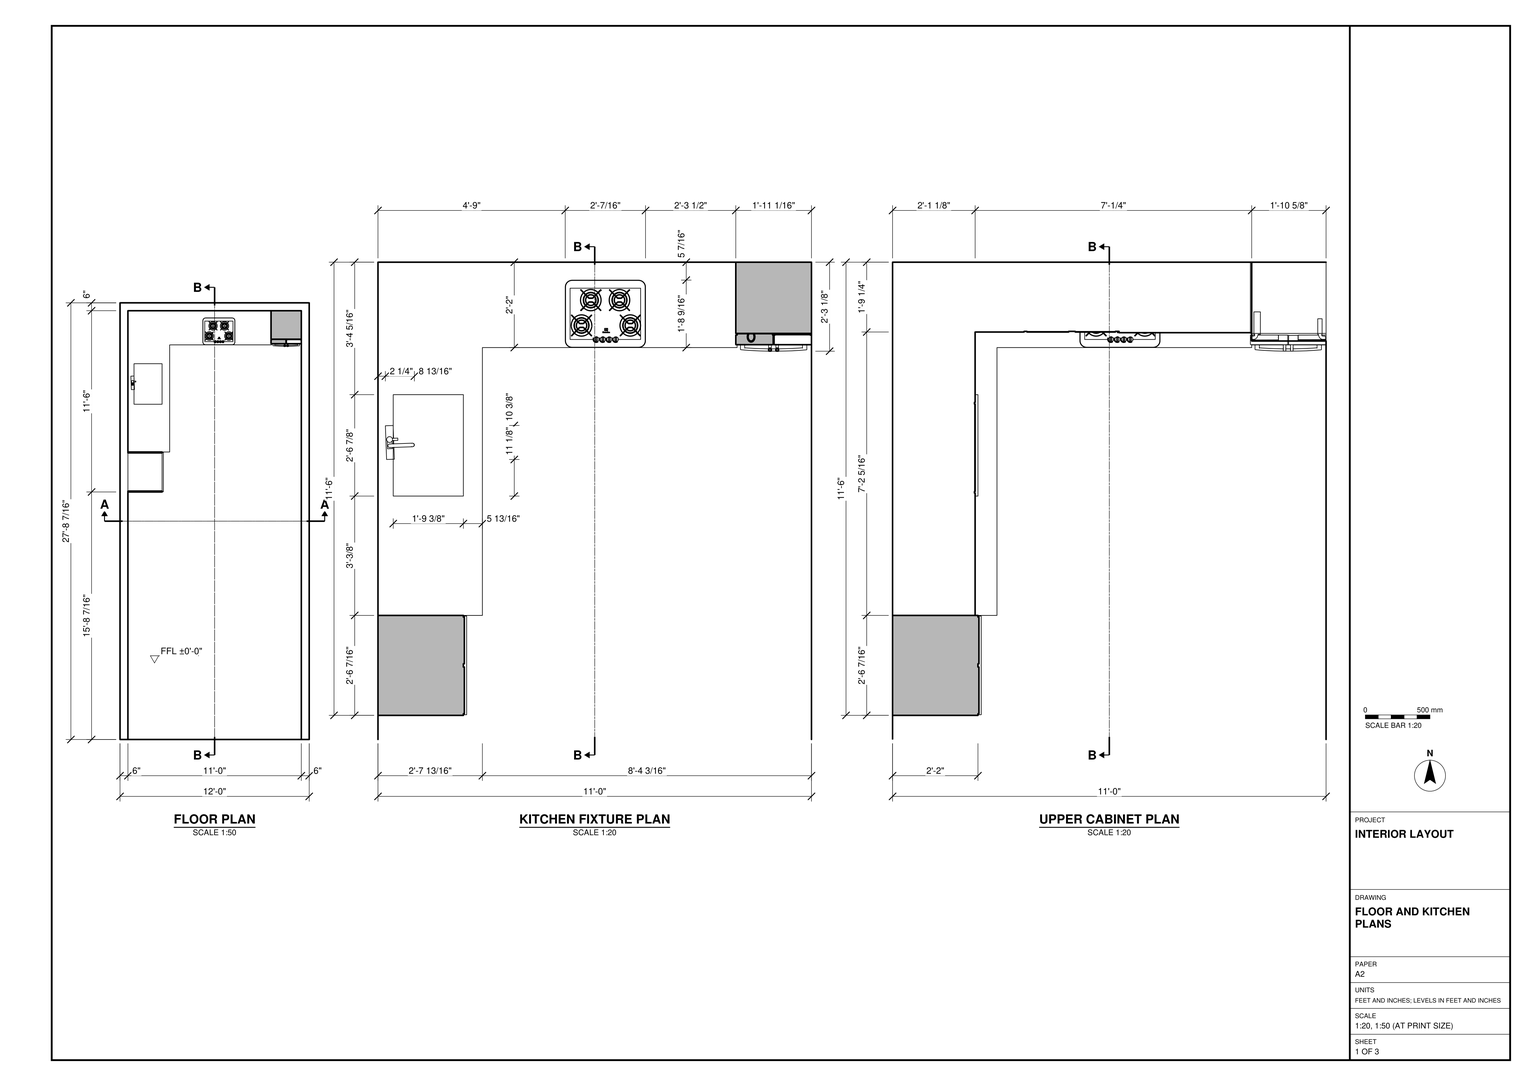
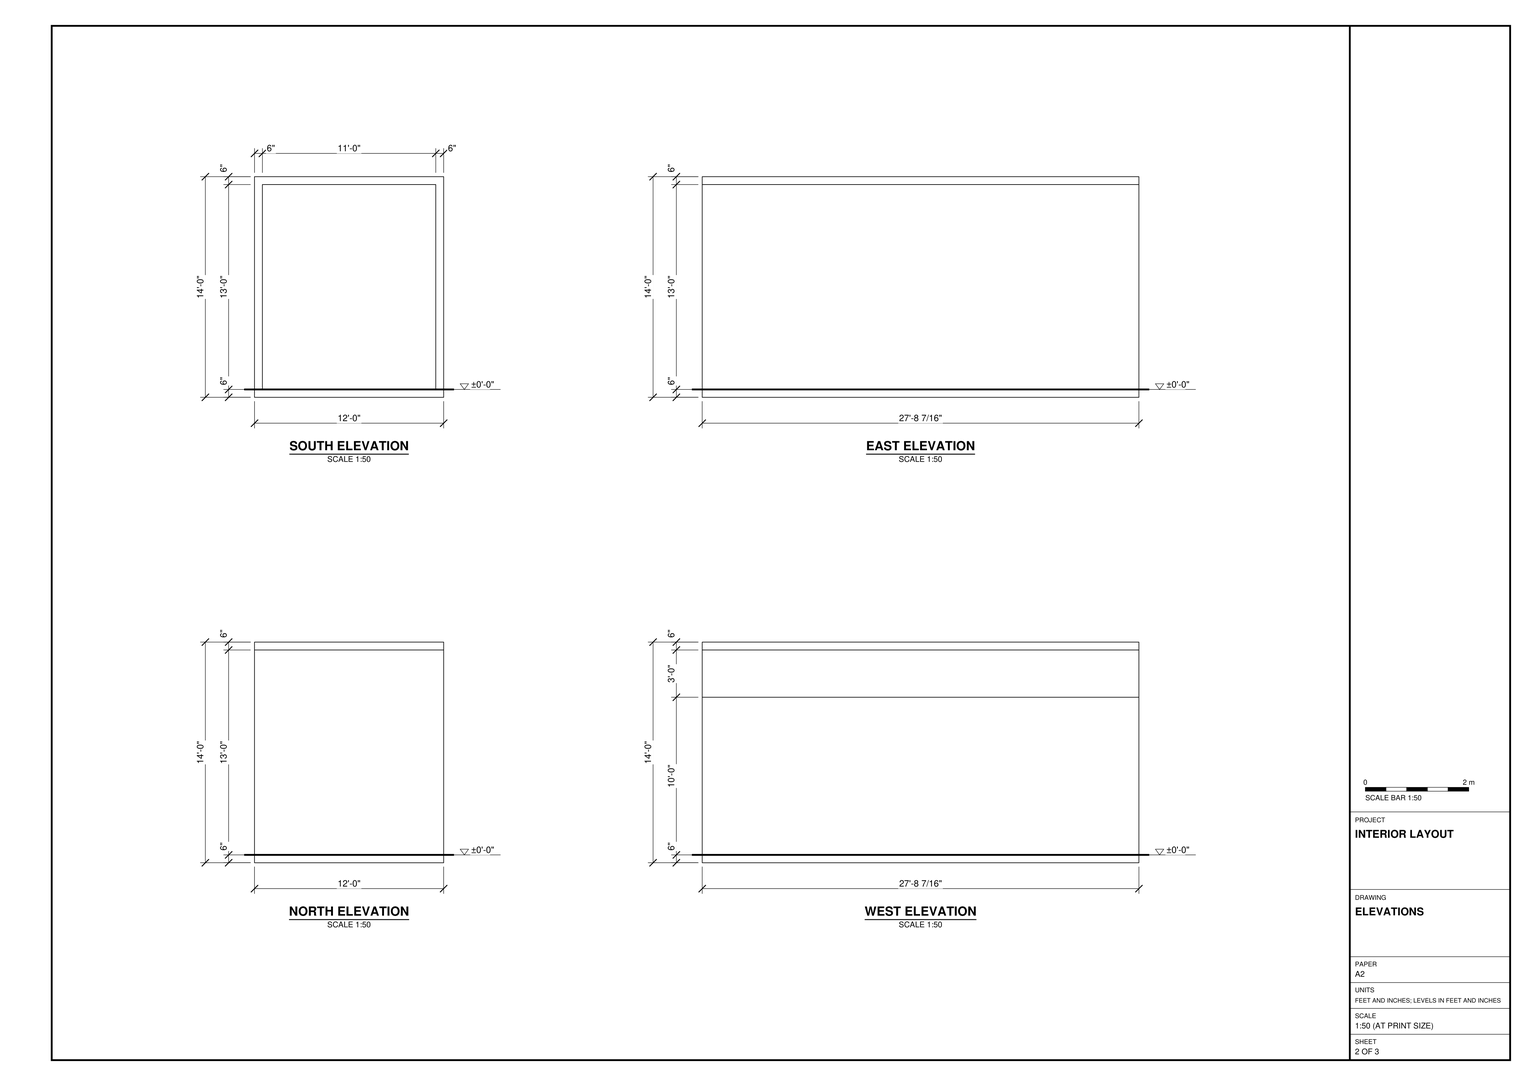
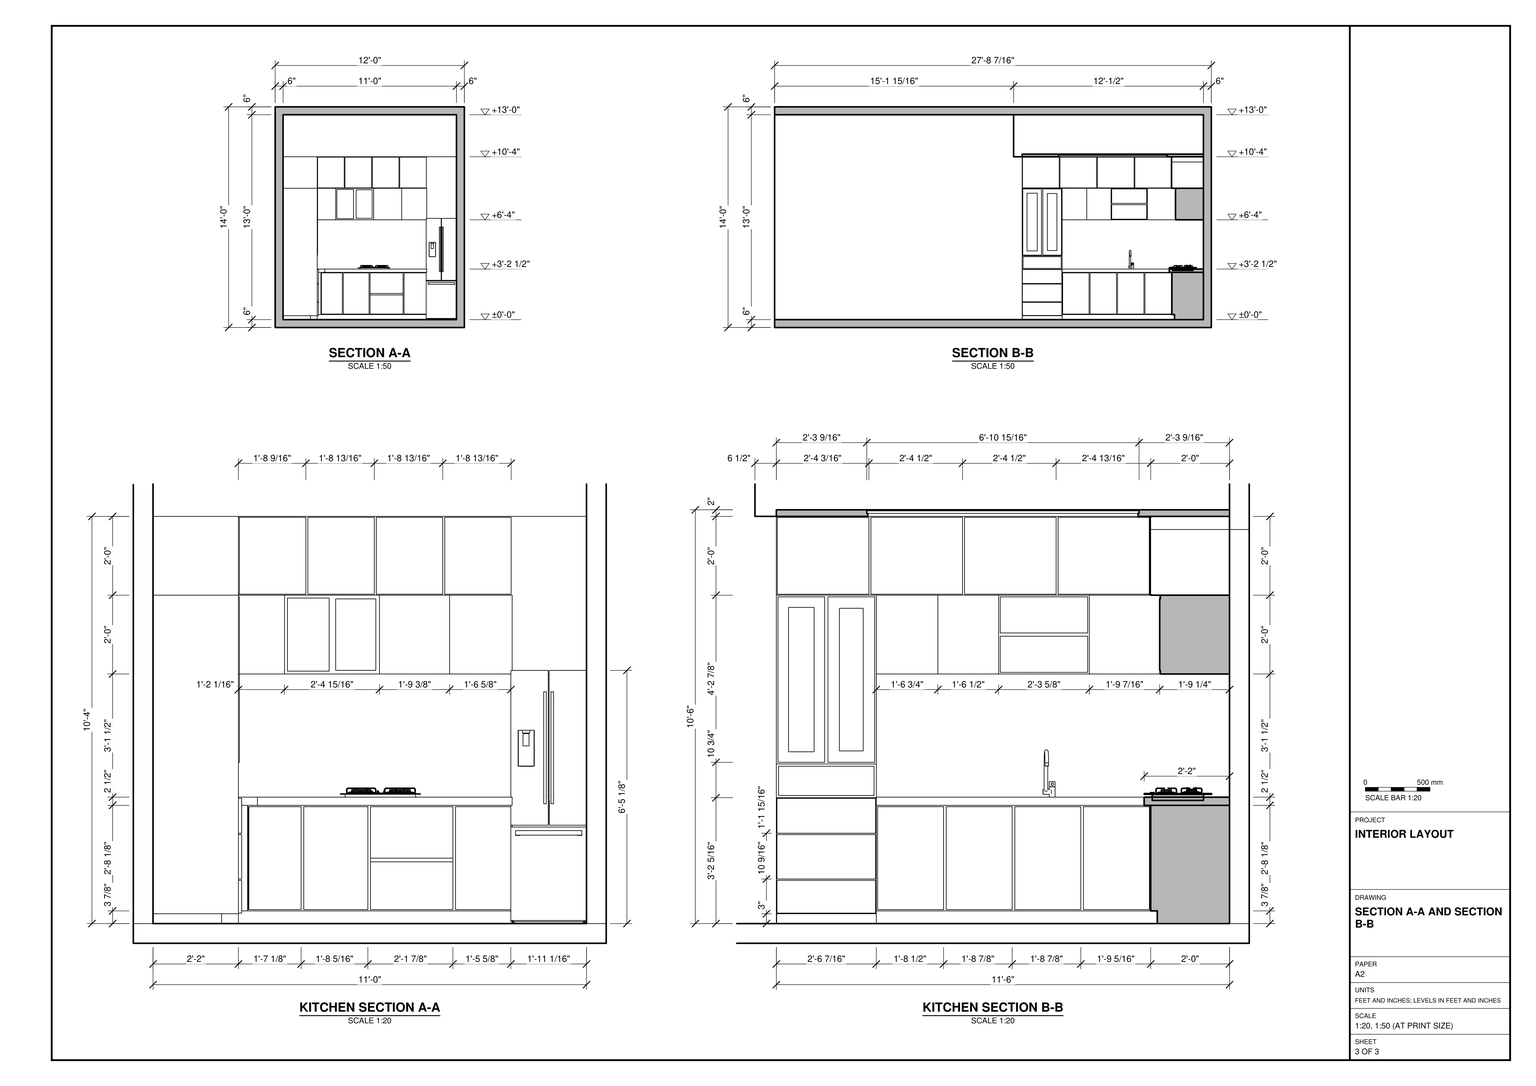
Build the interior in SketchUp using task_files/diagram_01.pdf. Work in feet and inches. Make the shell 12'-0" wide, 27'-8 7/16" long and 14'-0" high, with the finished floor at ±0'-0". Model the 6" side and north walls, the floor slab and the flat roof slab. Leave the south end open between the side walls, as shown in the floor plan and south elevation.

Fit the kitchen across the north end and along the west wall, leaving the floor to the south clear. Use the fixture plan to set out the worktop depths, the sink and tap on the west run, the cooktop on the north run and the refrigerator at the east end. Finish the west run with the tall storage unit. Use the upper cabinet plan for the overhead cabinet depths and the enlarged sections for the plinths, worktop height, door and drawer divisions, and two tiers of upper cabinets. Follow section B-B for the lowered soffit over the kitchen.

Keep the walls, slabs and roof as separate groups or components. Group each furniture or joinery piece separately and use components for repeated parts. Decor, loose items and appliances may be represented by any suitable library components. Save one SketchUp model as output_files/single_level_interior_with_an_l_shaped_kitchen.skp.

# SketchUp Ruby script. Lengths in inches.
U = 1.inch
M = Sketchup.active_model
def pt(a) = Geom::Point3d.new(a.map { |v| v * U })
def face(e, loops, mat)
  f = e.add_face(loops[0].map { |a| pt(a) })
  loops[1..].each { |l| e.add_face(l.map { |a| pt(a) }).erase! }
  f.material = f.back_material = mat if mat
  f
end
# faces: each face lists its corners as indices into pts; further lists are holes
def faces(e, pts, list, mat = nil) = list.each { |f| face(e, (f[0].is_a?(Array) ? f : [f]).map { |l| l.map { |i| pts[i] } }, mat) }
# xy, xz, yz: faces in a plane at the given z, y or x. An outline is a flat list of corners, or four numbers for a rectangle; further outlines are holes
def ring(l) = l.size == 4 ? [[l[0], l[1]], [l[2], l[1]], [l[2], l[3]], [l[0], l[3]]] : l.each_slice(2).to_a
def flat(e, list, mat, &to3) = list.each { |f| face(e, (f[0].is_a?(Array) ? f : [f]).map { |l| ring(l).map { |u, v| to3.(u, v) } }, mat) }
def xy(e, z, list, mat = nil) = flat(e, list, mat) { |x, y| [x, y, z] }
def xz(e, y, list, mat = nil) = flat(e, list, mat) { |x, z| [x, y, z] }
def yz(e, x, list, mat = nil) = flat(e, list, mat) { |y, z| [x, y, z] }
def lines(e, pts, list) = list.each { |a, b| e.add_line(pt(pts[a]), pt(pts[b])) }
# prism: a flat outline (further loops are holes) pulled along v
def prism(e, loops, v, mat = nil)
  f = face(e, loops, mat); d = Geom::Vector3d.new(v.map { |x| x * U })
  f.pushpull(f.normal.samedirection?(d) ? d.length : -d.length)
end
def box(e, o, s, mat = nil) = prism(e, [[o, [o[0] + s[0], o[1], o[2]], [o[0] + s[0], o[1] + s[1], o[2]], [o[0], o[1] + s[1], o[2]]]], [0, 0, s[2]], mat)
def at(x, y, z, deg = 0) = Geom::Transformation.translation(pt([x, y, z])) * Geom::Transformation.rotation(ORIGIN, Z_AXIS, deg.degrees)
def axes(o, x, y, z) = Geom::Transformation.new([*x, 0, *y, 0, *z, 0, *pt(o).to_a, 1])
def part(name) = M.definitions.add(name)
# library, detail: a bought-in or finely detailed component or shape, given as its bounding box
def library(name, o, s) = part(name).tap { |d| box(d.entities, o, s) }
def detail(e, o, s) = box(e.add_group.entities, o, s)
def put(e, d, t, mat = nil) = e.add_instance(d, t).tap { |i| i.material = mat if mat }
def group(e, t, mat = nil) = e.add_group.tap { |g| g.transformation = t; g.material = mat if mat }.entities
root = M.entities
M.materials.add("Emissive").color = [193, 160, 92]
M.materials.add("[0046_Gold]").color = [153, 128, 0]
M.materials.add("[0063_GreenYellow]").color = [65, 96, 17]
M.materials.add("[0130_Gainsboro]").color = [220, 220, 220]
M.materials.add("[0131_Silver]").color = [192, 192, 192]
M.materials.add("[0132_LightGray]").color = [169, 169, 169]
M.materials.add("[0133_Gray]").color = [128, 128, 128]
M.materials.add("[0134_DimGray]").color = [105, 105, 105]
M.materials.add("[0135_DarkGray]").color = [81, 81, 81]
M.materials.add("[0136_Charcoal]").color = [35, 35, 35]
M.materials.add("[Carrera Marble]").color = [207, 207, 207]
M.materials.add("[Marble Carrara Gold Floor Tile]").color = [224, 222, 216]
M.materials.add("[Translucent Glass Gray]").color = [128, 128, 128]
M.materials["[Translucent Glass Gray]"].alpha = 0.5
c1 = library("HELVEX-E-300-DX-EB",[0,0,0],[10.28,8.62,14.81])
c2 = library("Untitled",[22.625,2.94,30.74],[20.54,24.45,3.83])
c3 = library("B36CD50SNS_tradeCAD",[0,0,0],[35.84,30.35,69.65])
xy(root,-6,[[0,0,144,332.4375]])
xy(root,0,[[6,188.5625,26.875,188.5625,26.875,218.875,32,218.875,32,326.4375,6,326.4375],[32,304.4375,115.36,326.4375]])
xy(root,0,[[6,0,138,0,138,326.4375,115.36,326.4375,115.36,304.4375,32,304.4375,32,218.875,26.875,218.875,26.875,188.5625,6,188.5625]],"[Carrera Marble]")
xy(root,2.99,[[6,188.4375,26.875,188.5625]])
xy(root,2.99,[[26.875,188.4375,32,218.875]],"[0135_DarkGray]")
xy(root,3.19,[[32,188.64,33,218.68]],"[0135_DarkGray]")
xy(root,3.86,[[34.79,302.4375,115.36,304.4375]])
xy(root,3.86,[[32,218.875,34.79,304.4375]],"[0136_Charcoal]")
xy(root,4.26,[[35.19,302.24,51.1,302.4375],[51.9,302.24,71.43,302.4375],[72.23,302.24,97.32,302.4375],[98.12,302.24,114.96,302.4375]])
xy(root,4.26,[[34.79,219.28,34.99,239.37],[34.79,240.17,34.99,260.26],[34.79,261.06,34.99,281.15],[34.79,281.95,34.99,302.04]],"[0136_Charcoal]")
xy(root,13.17,[[32,188.64,33,218.68]],"[0135_DarkGray]")
xy(root,13.57,[[32,188.64,33,218.68]],"[0135_DarkGray]")
xy(root,18.8,[[72.23,302.24,97.32,302.4375]],"[0135_DarkGray]")
xy(root,19.93,[[72.23,302.24,97.32,302.4375]],"[0135_DarkGray]")
xy(root,27.11,[[32,188.64,33,218.68]],"[0135_DarkGray]")
xy(root,27.51,[[32,188.64,33,218.68]],"[0135_DarkGray]")
xy(root,35.6,[[34.79,219.28,34.99,239.37],[34.79,240.17,34.99,260.26],[34.79,261.06,34.99,281.15],[34.79,281.95,34.99,302.04],[35.19,302.24,37.79,302.4375],
  [72.23,302.24,97.32,302.4375],[98.12,302.24,114.96,302.4375]])
xy(root,35.6,[[37.79,302.24,51.1,302.4375],[51.9,302.24,71.43,302.4375]],"[0136_Charcoal]")
xy(root,36,[[6,218.875,6,326.4375,115.36,326.4375,115.36,302.4375,34.79,302.4375,34.79,218.875],[34.79,218.875,37.79,302.4375],[37.79,300.4375,115.36,302.4375]])
xy(root,36.4375,[[10.64,255.22,32.02,286.1]],"[0133_Gray]")
xy(root,38.13,[[32,188.64,33,218.68]],"[0135_DarkGray]")
xy(root,38.5,[[[6,218.875,37.79,218.875,37.79,300.4375,115.36,300.4375,115.36,326.4375,6,326.4375],[10.64,255.22,32.02,286.1]]],"[Marble Carrara Gold Floor Tile]")
xy(root,39.01,[[6,189.12,32,218.19]],"[0134_DimGray]")
xy(root,47.92,[[6,189.12,32,218.19]])
xy(root,49.1,[[32,188.9375,32.3,203.16],[32,204.16,32.3,218.375]])
xy(root,75.6875,[[115.36,302.4375,138,304.98]])
xy(root,75.6875,[[115.36,304.98,138,326.4375]],"[0135_DarkGray]")
xy(root,76,[[6,218.875,6,326.4375,115.36,326.4375,115.36,304.98,74.96,304.98,74.96,305.375,46.04,305.375,46.04,305.18,31.14,305.18,31.14,283.75,30.9375,283.75,30.9375,256.125,31.14,256.125,31.14,218.875]],"[0132_LightGray]")
xy(root,76.5,[[30.9375,256.625,31.14,283.25]])
xy(root,76.875,[[46.92,305.18,59.625,305.375]])
xy(root,77.12,[[61.62,305.18,73.84,305.375]])
xy(root,87.5,[[30.9375,256.625,31.14,283.25]],"[0134_DimGray]")
xy(root,88.5,[[30.9375,256.625,31.14,283.25]])
xy(root,98.88,[[61.62,305.18,73.84,305.375]])
xy(root,99.125,[[46.92,305.18,59.625,305.375]])
xy(root,99.5,[[30.9375,256.625,31.14,283.25]])
xy(root,99.5,[[32,188.9375,32.3,203.16],[32,204.16,32.3,218.375]],"[0131_Silver]")
xy(root,100,[[6,188.4375,32,218.875],[6,218.875,31.14,218.875,31.14,256.125,30.9375,256.125,30.9375,283.75,31.14,283.75,31.14,305.18,46.04,305.18,46.04,305.375,74.96,305.375,74.96,304.98,115.36,304.98,115.36,326.4375,6,326.4375],[31.14,218.875,32,237.625],[31.14,237.625,32,237.625,32,305.18,31.14,305.18,31.14,283.75,30.9375,283.75,30.9375,256.125,31.14,256.125],[32,302.4375,115.36,302.4375,115.36,304.98,74.96,304.98,74.96,305.375,46.04,305.375,46.04,305.18,32,305.18]])
xy(root,100.3,[[32,188.74,32.3,216.64],[32,217.24,32.3,218.875],[32,218.875,32.3,245.14],[32,245.74,32.3,273.64],[32,274.24,32.3,302.14],
  [32.3,302.14,52.54,302.4375],[53.14,302.14,73.38,302.4375],[73.98,302.14,94.22,302.4375],[94.82,302.14,115.06,302.4375]],"[0136_Charcoal]")
xy(root,123.7,[[32,188.74,32.3,216.64],[32,217.24,32.3,245.14],[32,245.74,32.3,273.64],[32,274.24,32.3,302.14],[32.3,302.14,52.54,302.4375],
  [53.14,302.14,73.38,302.4375],[73.98,302.14,94.22,302.4375],[94.82,302.14,115.06,302.4375]],"[0136_Charcoal]")
xy(root,124,[[6,181.9375,32,188.4375],[32,181.9375,138,188.4375]])
xy(root,124,[[6,188.4375,32,188.4375,32,302.4375,138,302.4375,138,326.4375,6,326.4375]],"[0135_DarkGray]")
xy(root,156,[[6,0,138,181.9375],[6,181.9375,138,326.4375]])
xy(root,162,[[0,0,144,332.4375]])
xz(root,0,[[[0,-6,144,162],[6,0,138,156]],[6,0,138,156]])
xz(root,181.9375,[[6,124,138,156]])
xz(root,188.4375,[[6,2.99,32,100],[6,100,32,124]],"[0135_DarkGray]")
xz(root,188.5625,[[6,0,26.875,2.99]],"[0135_DarkGray]")
xz(root,188.64,[[32,3.19,33,13.17],[32,13.57,33,27.11],[32,27.51,33,38.13]],"[0135_DarkGray]")
xz(root,188.74,[[32,100.3,32.3,123.7]],"[0136_Charcoal]")
xz(root,188.9375,[[32,49.1,32.3,99.5]],"[0136_Charcoal]")
xz(root,189.12,[[6,39.01,32,47.92]],"[0134_DimGray]")
xz(root,203.16,[[32,49.1,32.3,99.5]])
xz(root,204.16,[[32,49.1,32.3,99.5]],"[0136_Charcoal]")
xz(root,216.64,[[32,100.3,32.3,123.7]])
xz(root,217.24,[[32,100.3,32.3,123.7]],"[0136_Charcoal]")
xz(root,218.19,[[6,39.01,32,47.92]],"[0134_DimGray]")
xz(root,218.375,[[32,49.1,32.3,99.5]],"[0131_Silver]")
xz(root,218.68,[[32,3.19,33,3.86],[32,3.86,33,13.17],[32,13.57,33,27.11],[32,27.51,33,36],[32,36,33,38.13]],"[0135_DarkGray]")
xz(root,218.875,[[6,36,32,38.5],[6,38.5,32,76],[6,76,31.14,100],[31.14,76,32,100]])
xz(root,218.875,[[26.875,0,32,2.99],[32,3.86,34.79,36]],"[0134_DimGray]")
xz(root,218.875,[[32,36,37.79,38.5]],"[Marble Carrara Gold Floor Tile]")
xz(root,219.28,[[34.79,4.26,34.99,35.6]],"[0136_Charcoal]")
xz(root,239.37,[[34.79,4.26,34.99,35.6]])
xz(root,240.17,[[34.79,4.26,34.99,35.6]],"[0136_Charcoal]")
xz(root,245.14,[[32,100.3,32.3,123.7]],"[0136_Charcoal]")
xz(root,245.74,[[32,100.3,32.3,123.7]],"[0136_Charcoal]")
xz(root,255.22,[[10.64,36.4375,32.02,38.5]])
xz(root,256.125,[[30.9375,76,31.14,100]])
xz(root,256.625,[[30.9375,76.5,31.14,87.5],[30.9375,88.5,31.14,99.5]],"[0134_DimGray]")
xz(root,260.26,[[34.79,4.26,34.99,35.6]])
xz(root,261.06,[[34.79,4.26,34.99,35.6]],"[0136_Charcoal]")
xz(root,273.64,[[32,100.3,32.3,123.7]],"[0136_Charcoal]")
xz(root,274.24,[[32,100.3,32.3,123.7]],"[0136_Charcoal]")
xz(root,281.15,[[34.79,4.26,34.99,35.6]])
xz(root,281.95,[[34.79,4.26,34.99,35.6]],"[0136_Charcoal]")
xz(root,283.25,[[30.9375,76.5,31.14,87.5],[30.9375,88.5,31.14,99.5]],"[0134_DimGray]")
xz(root,283.75,[[30.9375,76,31.14,100]],"[0134_DimGray]")
xz(root,286.1,[[10.64,36.4375,32.02,38.5]],"[0133_Gray]")
xz(root,300.4375,[[37.79,36,115.36,38.5]],"[Marble Carrara Gold Floor Tile]")
xz(root,302.04,[[34.79,4.26,34.99,35.6]])
xz(root,302.14,[[32,100.3,32.3,123.7]])
xz(root,302.14,[[32.3,100.3,52.54,123.7],[53.14,100.3,73.38,123.7],[73.98,100.3,94.22,123.7],[94.82,100.3,115.06,123.7]],"[0135_DarkGray]")
xz(root,302.24,[[35.19,4.26,51.1,35.6],[51.9,4.26,71.43,35.6],[72.23,4.26,97.32,18.8],[98.12,4.26,114.96,35.6],[72.23,19.93,97.32,35.6]],"[0135_DarkGray]")
xz(root,302.4375,[[72.23,18.8,97.32,19.93]],"[0135_DarkGray]")
xz(root,302.4375,[[[34.79,3.86,115.36,36],[72.23,4.26,97.32,35.6],[51.9,4.26,71.43,35.6],[98.12,4.26,114.96,35.6],[35.19,4.26,51.1,35.6]],[[115.36,75.6875,138,75.6875,138,124,32,124,32,100,115.36,100],[53.14,100.3,73.38,123.7],[32.3,100.3,52.54,123.7],[94.82,100.3,115.06,123.7],[73.98,100.3,94.22,123.7]]],"[0136_Charcoal]")
xz(root,304.4375,[[32,0,115.36,3.86]],"[0134_DimGray]")
xz(root,304.98,[[74.96,76,96.3125,100],[96.3125,76,115.36,100]],"[0132_LightGray]")
xz(root,305.18,[[31.14,76,46.04,100]],"[0132_LightGray]")
xz(root,305.18,[[46.92,76.875,59.625,99.125],[61.62,77.12,73.84,98.88]],"[Translucent Glass Gray]")
xz(root,305.375,[[[46.04,76,74.96,100],[46.92,76.875,59.625,99.125],[61.62,77.12,73.84,98.88]]],"[0134_DimGray]")
xz(root,326.4375,[[6,0,115.36,36],[6,36,115.36,38.5],[115.36,75.6875,138,75.6875,138,124,6,124,6,100,115.36,100]])
xz(root,326.4375,[[6,76,115.36,100]],"Emissive")
xz(root,326.4375,[[115.36,0,138,0,138,75.6875,115.36,75.6875,115.36,76,6,76,6,38.5,115.36,38.5]],"[0046_Gold]")
xz(root,326.4375,[[6,124,138,156]],"[0063_GreenYellow]")
xz(root,332.4375,[[0,-6,144,0],[0,0,144,156],[0,156,144,162]])
yz(root,0,[[0,-6,332.4375,0],[0,120,332.4375,156],[0,156,332.4375,162]])
yz(root,0,[[0,0,332.4375,120]],"[0134_DimGray]")
yz(root,6,[[0,0,188.4375,0,188.4375,124,181.9375,124,181.9375,156,0,156],[188.4375,0,188.5625,2.99],[218.875,0,326.4375,36],[218.875,36,326.4375,38.5],[188.4375,100,326.4375,120],
  [188.4375,120,326.4375,124]])
yz(root,6,[[[188.5625,0,218.875,0,218.875,100,188.4375,100,188.4375,2.99,188.5625,2.99],[189.12,39.01,218.19,47.92]],[218.875,76,326.4375,100]],"Emissive")
yz(root,6,[[218.875,38.5,326.4375,76]],"[0046_Gold]")
yz(root,6,[[181.9375,124,326.4375,156]],"[0063_GreenYellow]")
yz(root,10.64,[[255.22,36.4375,286.1,38.5]],"[0133_Gray]")
yz(root,26.875,[[188.5625,0,218.875,2.99]],"[0135_DarkGray]")
yz(root,30.9375,[[[256.125,76,283.75,100],[256.625,88.5,283.25,99.5],[256.625,76.5,283.25,87.5]]],"[0134_DimGray]")
yz(root,31.14,[[218.875,76,237.625,100],[237.625,76,256.125,100],[283.75,76,305.18,100]],"[0130_Gainsboro]")
yz(root,31.14,[[256.625,76.5,283.25,87.5],[256.625,88.5,283.25,99.5]],"[Translucent Glass Gray]")
yz(root,32,[[188.64,27.51,218.68,38.13]])
yz(root,32,[[[188.4375,48.6,218.875,100],[188.9375,49.1,203.16,99.5],[204.16,49.1,218.375,99.5]]],"[0131_Silver]")
yz(root,32,[[218.875,0,304.4375,3.86]],"[0134_DimGray]")
yz(root,32,[[[188.4375,2.99,218.875,2.99,218.875,38.33,218.68,38.13,218.68,27.51,188.64,27.51,188.64,38.13,188.4375,38.13],[188.64,13.57,218.68,27.11],[188.64,3.19,218.68,13.17]],[188.4375,38.13,218.68,38.13,218.875,38.33,188.4375,38.33],[[188.4375,38.33,218.875,48.6],[189.12,39.01,218.19,47.92]],[[188.4375,100,302.4375,124],[217.24,100.3,245.14,123.7],[188.74,100.3,216.64,123.7],[245.74,100.3,273.64,123.7],[274.24,100.3,302.14,123.7]]],"[0136_Charcoal]")
yz(root,32.02,[[255.22,36.4375,286.1,38.5]])
yz(root,32.3,[[302.14,100.3,302.4375,123.7]])
yz(root,32.3,[[[188.9375,49.1,203.16,99.5],[192.15,52.3125,199.94,96.29]],[[204.16,49.1,218.375,99.5],[207.63,52.58,214.9,96.02]]],"[0131_Silver]")
yz(root,32.3,[[188.74,100.3,216.64,123.7],[217.24,100.3,245.14,123.7],[245.74,100.3,273.64,123.7],[274.24,100.3,302.14,123.7]],"[0135_DarkGray]")
yz(root,32.3,[[192.15,52.3125,199.94,96.29],[207.63,52.58,214.9,96.02]],"[Translucent Glass Gray]")
yz(root,33,[[188.64,3.19,218.68,13.17],[188.64,13.57,218.68,27.11],[188.64,27.51,218.68,38.13]],"[0135_DarkGray]")
yz(root,34.79,[[[218.875,3.86,302.4375,36],[219.28,4.26,239.37,35.6],[281.95,4.26,302.04,35.6],[261.06,4.26,281.15,35.6],[240.17,4.26,260.26,35.6]]],"[0136_Charcoal]")
yz(root,34.99,[[219.28,4.26,239.37,35.6],[240.17,4.26,260.26,35.6],[261.06,4.26,281.15,35.6],[281.95,4.26,302.04,35.6]],"[0135_DarkGray]")
yz(root,35.19,[[302.24,4.26,302.4375,35.6]])
yz(root,37.79,[[218.875,36,300.4375,38.5]],"[Marble Carrara Gold Floor Tile]")
yz(root,46.04,[[305.18,76,305.375,100]])
yz(root,46.92,[[305.18,76.875,305.375,99.125]])
yz(root,51.1,[[302.24,4.26,302.4375,35.6]],"[0136_Charcoal]")
yz(root,51.9,[[302.24,4.26,302.4375,35.6]],"[0136_Charcoal]")
yz(root,52.54,[[302.14,100.3,302.4375,123.7]],"[0136_Charcoal]")
yz(root,53.14,[[302.14,100.3,302.4375,123.7]])
yz(root,59.625,[[305.18,76.875,305.375,99.125]])
yz(root,61.62,[[305.18,77.12,305.375,98.88]])
yz(root,71.43,[[302.24,4.26,302.4375,35.6]])
yz(root,72.23,[[302.24,4.26,302.4375,18.8],[302.24,19.93,302.4375,35.6]])
yz(root,73.38,[[302.14,100.3,302.4375,123.7]],"[0136_Charcoal]")
yz(root,73.84,[[305.18,77.12,305.375,98.88]])
yz(root,73.98,[[302.14,100.3,302.4375,123.7]],"[0136_Charcoal]")
yz(root,74.96,[[304.98,76,305.375,100]])
yz(root,94.22,[[302.14,100.3,302.4375,123.7]],"[0136_Charcoal]")
yz(root,94.82,[[302.14,100.3,302.4375,123.7]],"[0136_Charcoal]")
yz(root,97.32,[[302.24,4.26,302.4375,18.8],[302.24,19.93,302.4375,35.6]])
yz(root,98.12,[[302.24,4.26,302.4375,35.6]])
yz(root,114.96,[[302.24,4.26,302.4375,35.6]])
yz(root,115.06,[[302.14,100.3,302.4375,123.7]],"[0136_Charcoal]")
yz(root,115.36,[[302.4375,75.6875,304.98,100]])
yz(root,115.36,[[304.98,76,326.4375,100]],"[0130_Gainsboro]")
yz(root,115.36,[[304.4375,0,326.4375,3.86],[302.4375,3.86,326.4375,36],[304.98,75.6875,326.4375,76]],"[0135_DarkGray]")
yz(root,115.36,[[300.4375,36,326.4375,38.5]],"[Marble Carrara Gold Floor Tile]")
yz(root,138,[[0,0,0,156,326.4375,156,326.4375,124,302.4375,124,302.4375,75.6875,326.4375,75.6875,326.4375,0]])
yz(root,144,[[0,-6,332.4375,0],[0,0,332.4375,156],[0,156,332.4375,162]])
put(root,c1,at(17.24,266.67,38.11,92.083))
put(root,c2,at(60.08,343.61,6.77,-90))
put(root,c3,axes([114.96,299.33,0],[0.64294,0,0],[0,0.89294,0],[0,0,1.107]))
g1 = group(root,at(6,188.4375,124))
xy(g1,0,[[[0,0,132,138],[27.85,27.85,104.15,110.15]]])
xy(g1,0.91,[[27.55,27.55,104.15,27.85],[104.15,27.55,104.45,110.15],[27.55,27.85,27.85,110.15],[27.55,110.15,104.45,110.45]])
xy(g1,1.8125,[[27.55,27.55,104.45,110.45]])
xy(g1,2,[[0,0,132,138]])
xz(g1,0,[[0,0,132,2]])
xz(g1,27.55,[[27.55,0.91,104.45,1.8125]],"Emissive")
xz(g1,27.85,[[27.85,0,104.15,0.91]])
xz(g1,110.15,[[27.85,0,104.15,0.91]])
xz(g1,110.45,[[27.55,0.91,104.45,1.8125]],"Emissive")
xz(g1,138,[[0,0,132,2]])
yz(g1,0,[[0,0,138,2]])
yz(g1,27.55,[[27.55,0.91,110.45,1.8125]],"Emissive")
yz(g1,27.85,[[27.85,0,110.15,0.91]])
yz(g1,104.15,[[27.85,0,110.15,0.91]])
yz(g1,104.45,[[27.55,0.91,110.45,1.8125]],"Emissive")
yz(g1,132,[[0,0,138,2]])
